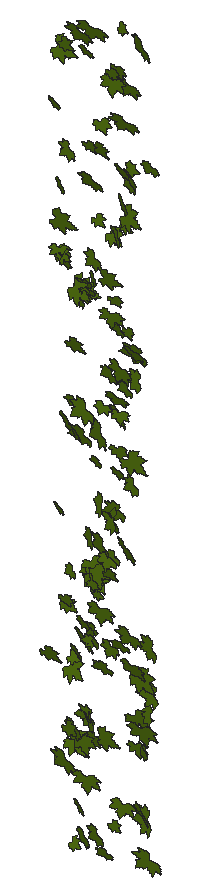
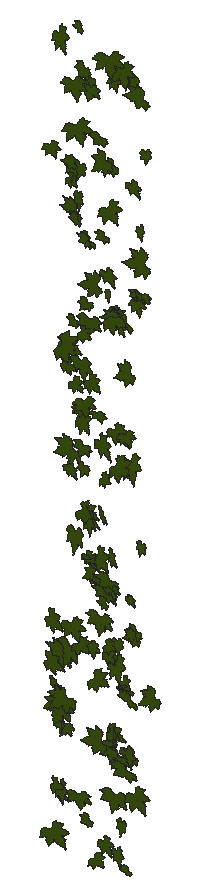
# SketchUp Ruby script. Lengths in inches.
U = 1.inch
M = Sketchup.active_model
def pt(a) = Geom::Point3d.new(a.map { |v| v * U })
def face(e, loops, mat)
  f = e.add_face(loops[0].map { |a| pt(a) })
  loops[1..].each { |l| e.add_face(l.map { |a| pt(a) }).erase! }
  f.material = f.back_material = mat if mat
  f
end
# faces: each face lists its corners as indices into pts; further lists are holes
def faces(e, pts, list, mat = nil) = list.each { |f| face(e, (f[0].is_a?(Array) ? f : [f]).map { |l| l.map { |i| pts[i] } }, mat) }
# xy, xz, yz: faces in a plane at the given z, y or x. An outline is a flat list of corners, or four numbers for a rectangle; further outlines are holes
def ring(l) = l.size == 4 ? [[l[0], l[1]], [l[2], l[1]], [l[2], l[3]], [l[0], l[3]]] : l.each_slice(2).to_a
def flat(e, list, mat, &to3) = list.each { |f| face(e, (f[0].is_a?(Array) ? f : [f]).map { |l| ring(l).map { |u, v| to3.(u, v) } }, mat) }
def xy(e, z, list, mat = nil) = flat(e, list, mat) { |x, y| [x, y, z] }
def xz(e, y, list, mat = nil) = flat(e, list, mat) { |x, z| [x, y, z] }
def yz(e, x, list, mat = nil) = flat(e, list, mat) { |y, z| [x, y, z] }
def lines(e, pts, list) = list.each { |a, b| e.add_line(pt(pts[a]), pt(pts[b])) }
# prism: a flat outline (further loops are holes) pulled along v
def prism(e, loops, v, mat = nil)
  f = face(e, loops, mat); d = Geom::Vector3d.new(v.map { |x| x * U })
  f.pushpull(f.normal.samedirection?(d) ? d.length : -d.length)
end
def box(e, o, s, mat = nil) = prism(e, [[o, [o[0] + s[0], o[1], o[2]], [o[0] + s[0], o[1] + s[1], o[2]], [o[0], o[1] + s[1], o[2]]]], [0, 0, s[2]], mat)
def at(x, y, z, deg = 0) = Geom::Transformation.translation(pt([x, y, z])) * Geom::Transformation.rotation(ORIGIN, Z_AXIS, deg.degrees)
def axes(o, x, y, z) = Geom::Transformation.new([*x, 0, *y, 0, *z, 0, *pt(o).to_a, 1])
def part(name) = M.definitions.add(name)
# library, detail: a bought-in or finely detailed component or shape, given as its bounding box
def library(name, o, s) = part(name).tap { |d| box(d.entities, o, s) }
def detail(e, o, s) = box(e.add_group.entities, o, s)
def put(e, d, t, mat = nil) = e.add_instance(d, t).tap { |i| i.material = mat if mat }
def group(e, t, mat = nil) = e.add_group.tap { |g| g.transformation = t; g.material = mat if mat }.entities
root = M.entities
M.materials.add("[Vegetation Blur 03]").color = [83, 114, 18]
c1 = part("ivy")
xy(c1.entities,0,[[0.782,0,0.786,0,0.787,0.005,0.789,0.009,0.821,0.072,0.875,0.147,1.001,0.272,1.073,0.331,1.137,0.363,1.178,0.379,1.223,0.384,1.272,0.383,1.311,0.374,1.36,0.355,1.399,0.334,1.491,0.285,1.541,0.244,1.583,0.199,1.617,0.15,1.64,0.128,1.662,0.115,1.717,0.105,1.745,0.093,1.784,0.054,1.819,0.057,1.854,0.064,1.882,0.075,1.896,0.074,1.91,0.071,1.937,0.063,1.964,0.053,1.99,0.038,2.016,0.015,2.034,0.002,2.04,0,2.038,0.003,2.036,0.007,2.033,0.038,2.036,0.068,2.045,0.1,2.055,0.116,2.064,0.123,2.077,0.129,2.088,0.129,2.106,0.132,2.118,0.13,2.179,0.132,2.207,0.133,2.225,0.133,2.242,0.138,2.22,0.162,2.207,0.186,2.206,0.213,2.212,0.236,2.228,0.262,2.247,0.274,2.298,0.283,2.355,0.294,2.37,0.296,2.376,0.295,2.377,0.3,2.377,0.303,2.385,0.329,2.411,0.37,2.426,0.392,2.449,0.407,2.511,0.426,2.561,0.444,2.619,0.466,2.589,0.469,2.561,0.476,2.501,0.5,2.449,0.516,2.424,0.523,2.401,0.535,2.377,0.556,2.372,0.568,2.36,0.575,2.268,0.586,2.225,0.592,2.207,0.599,2.194,0.61,2.143,0.65,2.13,0.664,2.122,0.682,2.123,0.7,2.13,0.719,2.148,0.75,2.17,0.781,2.195,0.807,2.221,0.828,2.284,0.874,2.291,0.88,2.288,0.887,2.276,0.9,2.267,0.916,2.265,0.933,2.273,0.967,2.292,1.002,2.313,1.03,2.334,1.054,2.348,1.067,2.358,1.074,2.363,1.076,2.362,1.081,2.35,1.094,2.347,1.11,2.35,1.143,2.359,1.18,2.385,1.254,2.415,1.324,2.448,1.393,2.45,1.4,2.446,1.398,2.44,1.394,2.427,1.383,2.402,1.36,2.376,1.339,2.345,1.324,2.305,1.309,2.282,1.303,2.273,1.306,2.245,1.294,2.212,1.287,2.187,1.291,2.163,1.301,2.142,1.316,2.134,1.327,2.124,1.325,2.09,1.292,2.053,1.259,2.014,1.234,1.973,1.215,1.954,1.21,1.931,1.208,1.909,1.212,1.893,1.22,1.879,1.233,1.872,1.248,1.867,1.281,1.864,1.319,1.821,1.258,1.773,1.197,1.726,1.141,1.698,1.121,1.679,1.116,1.666,1.117,1.647,1.122,1.632,1.129,1.62,1.141,1.617,1.154,1.617,1.219,1.621,1.254,1.623,1.268,1.623,1.281,1.618,1.314,1.606,1.346,1.603,1.375,1.607,1.403,1.603,1.467,1.599,1.499,1.605,1.525,1.614,1.552,1.629,1.577,1.635,1.589,1.629,1.587,1.618,1.582,1.596,1.566,1.581,1.556,1.568,1.552,1.557,1.55,1.545,1.553,1.531,1.562,1.522,1.572,1.504,1.591,1.486,1.611,1.474,1.631,1.457,1.666,1.455,1.684,1.457,1.698,1.452,1.715,1.444,1.728,1.424,1.754,1.419,1.772,1.423,1.786,1.434,1.819,1.444,1.848,1.446,1.855,1.44,1.861,1.43,1.867,1.386,1.904,1.349,1.948,1.326,1.973,1.31,1.995,1.288,2.048,1.284,2.153,1.287,2.254,1.284,2.255,1.282,2.253,1.278,2.247,1.274,2.237,1.266,2.216,1.226,2.125,1.208,2.076,1.184,2.033,1.155,1.984,1.135,1.942,1.111,1.899,1.083,1.861,1.053,1.85,1.059,1.83,1.061,1.809,1.056,1.79,1.049,1.767,1.04,1.749,1.018,1.733,0.994,1.726,0.942,1.734,0.95,1.6875,0.944,1.645,0.932,1.608,0.911,1.585,0.881,1.58,0.854,1.582,0.828,1.588,0.785,1.618,0.773,1.625,0.775,1.614,0.779,1.598,0.796,1.502,0.818,1.402,0.861,1.283,0.882,1.224,0.894,1.174,0.892,1.148,0.886,1.123,0.881,1.107,0.872,1.099,0.849,1.094,0.818,1.092,0.789,1.098,0.762,1.107,0.753,1.113,0.721,1.139,0.698,1.163,0.678,1.194,0.665,1.224,0.628,1.28,0.612,1.312,0.606,1.327,0.606,1.314,0.599,1.282,0.594,1.267,0.581,1.256,0.544,1.245,0.512,1.244,0.473,1.249,0.444,1.256,0.382,1.288,0.339,1.306,0.324,1.316,0.317,1.324,0.309,1.326,0.27,1.314,0.227,1.313,0.185,1.3125,0.152,1.317,0.122,1.328,0.092,1.345,0.073,1.353,0.079,1.338,0.092,1.308,0.117,1.249,0.13,1.215,0.139,1.164,0.147,1.148,0.157,1.136,0.163,1.122,0.174,1.086,0.177,1.067,0.182,1.054,0.186,1.043,0.191,1.038,0.211,1.028,0.237,1.005,0.25,0.974,0.253,0.96,0.25,0.944,0.242,0.914,0.243,0.906,0.249,0.902,0.26,0.894,0.289,0.88,0.307,0.873,0.322,0.862,0.364,0.799,0.403,0.738,0.431,0.709,0.439,0.691,0.441,0.678,0.4375,0.66,0.428,0.645,0.394,0.623,0.303,0.594,0.255,0.581,0.214,0.577,0.179,0.573,0.173,0.568,0.175,0.561,0.167,0.55,0.141,0.523,0.113,0.503,0.077,0.49,0.045,0.486,0.026,0.485,0.019,0.486,0.011,0.483,0,0.471,0.014,0.467,0.044,0.455,0.058,0.447,0.07,0.438,0.097,0.411,0.125,0.394,0.158,0.377,0.174,0.366,0.182,0.359,0.185,0.361,0.242,0.331,0.253,0.316,0.258,0.303,0.262,0.283,0.274,0.278,0.308,0.274,0.341,0.252,0.366,0.226,0.366,0.222,0.37,0.22,0.38,0.221,0.395,0.221,0.425,0.216,0.45,0.207,0.465,0.192,0.473,0.178,0.484,0.15,0.489,0.116,0.483,0.089,0.468,0.058,0.45,0.035,0.435,0.018,0.429,0.011,0.434,0.012,0.438,0.014,0.469,0.019,0.542,0.016,0.581,0.015,0.612,0.027,0.68,0.055,0.696,0.057,0.712,0.052,0.73,0.045,0.741,0.036,0.766,0.014]])
put(root,c1,axes([17.67,173.7,15.6],[0.33482,-0.12296,0.29954],[0.37174,0.13576,-0.26801],[0.00918,-1.01326,-0.07226]),"[Vegetation Blur 03]")
put(root,c1,axes([18.34,173.7,44.47],[0.29211,-0.05666,-0.12031],[-0.1385,0.15286,-0.23529],[-0.05752,-0.65573,-0.04445]),"[Vegetation Blur 03]")
put(root,c1,axes([18.82,173.7,40.44],[0.23798,-0.09799,-0.20106],[-0.2294,0.19812,-0.19604],[-0.10166,-0.67644,-0.02829]),"[Vegetation Blur 03]")
put(root,c1,axes([18.85,173.7,11.16],[0.44315,0.00145,-0.39097],[-0.47521,0.17095,-0.35867],[-0.06051,-1.33197,-0.04646]),"[Vegetation Blur 03]")
put(root,c1,axes([18.59,173.7,23.7],[0.31001,-0.14403,-0.03677],[-0.03088,0.13304,-0.25536],[-0.0773,-0.63077,-0.04546]),"[Vegetation Blur 03]")
put(root,c1,axes([18.78,173.7,36.65],[0.35037,-0.01321,-0.20166],[-0.24181,0.16441,-0.28153],[-0.0512,-0.86678,-0.05033]),"[Vegetation Blur 03]")
put(root,c1,axes([18.3,173.7,36.83],[0.4392,0.07424,0.06802],[0.08567,-0.05755,-0.35857],[0.03015,-0.91812,0.02798]),"[Vegetation Blur 03]")
put(root,c1,axes([19.05,173.7,28.47],[0.46716,-0.062,-0.38996],[-0.44887,0.42109,-0.3687],[-0.16652,-1.30905,-0.10013]),"[Vegetation Blur 03]")
put(root,c1,axes([18.33,173.7,46.5],[0.13182,0.09274,0.49871],[0.61259,0.00582,-0.10802],[0.01227,-1.28635,0.03547]),"[Vegetation Blur 03]")
put(root,c1,axes([18.61,173.7,36.14],[0.09631,0.08819,0.32844],[0.40359,-0.08421,-0.07527],[-0.03009,-0.84734,0.04167]),"[Vegetation Blur 03]")
put(root,c1,axes([18.33,173.7,37.74],[0.17934,-0.09894,0.51265],[0.6295,0.08025,-0.14425],[0.02442,-1.34184,-0.04643]),"[Vegetation Blur 03]")
put(root,c1,axes([19.26,173.7,42.62],[0.34594,-0.11487,-0.25725],[-0.31497,0.04827,-0.28551],[-0.05712,-0.96184,0.01639]),"[Vegetation Blur 03]")
put(root,c1,axes([18.78,173.7,18.89],[0.3213,-0.06644,0.14929],[0.18483,0.03966,-0.26218],[-0.01845,-0.75978,-0.02674]),"[Vegetation Blur 03]")
put(root,c1,axes([18.79,173.7,47.24],[0.18668,-0.06069,0.28857],[0.35478,0.02187,-0.15215],[-0.00434,-0.8225,-0.02534]),"[Vegetation Blur 03]")
put(root,c1,axes([18.86,173.7,18.36],[0.19136,0.01715,0.31471],[0.38568,-0.01715,-0.15606],[-0.00376,-0.88569,0.00911]),"[Vegetation Blur 03]")
put(root,c1,axes([19.41,173.7,29.49],[0.29858,0.09929,-0.17499],[-0.21887,0.06675,-0.24279],[0.01995,-0.75348,-0.04457]),"[Vegetation Blur 03]")
put(root,c1,axes([19.55,173.7,20.86],[0.2154,-0.10325,-0.19292],[-0.23671,0.04089,-0.17948],[-0.04859,-0.65681,0.01915]),"[Vegetation Blur 03]")
put(root,c1,axes([19.8,173.7,16.61],[0.12889,0.05373,-0.25764],[-0.31029,0.16238,-0.09807],[-0.06367,-0.68262,-0.04361]),"[Vegetation Blur 03]")
put(root,c1,axes([19.43,173.7,12.93],[0.42245,-0.13873,-0.23601],[-0.28027,0.15555,-0.34853],[-0.09809,-1.04193,-0.02061]),"[Vegetation Blur 03]")
put(root,c1,axes([19.27,173.7,15.65],[0.07011,0.12287,0.23012],[0.28735,0.0166,-0.05971],[0.0224,-0.59768,0.04565]),"[Vegetation Blur 03]")
put(root,c1,axes([18.99,173.7,12.1],[0.22931,-0.05412,0.29769],[0.36487,-0.02596,-0.18795],[-0.02469,-0.88622,-0.01267]),"[Vegetation Blur 03]")
put(root,c1,axes([20.1,173.7,28.09],[0.19085,0.16255,-0.44019],[-0.54494,0.0863,-0.15236],[-0.01363,-1.17416,-0.07214]),"[Vegetation Blur 03]")
put(root,c1,axes([19.43,173.7,48.74],[0.51903,0.05216,-0.26245],[-0.32095,0.20906,-0.41624],[-0.03231,-1.23893,-0.08129]),"[Vegetation Blur 03]")
put(root,c1,axes([19.39,173.7,6.15],[0.08845,0.08211,0.23234],[0.28731,-0.04554,-0.07032],[-0.00952,-0.61175,0.03642]),"[Vegetation Blur 03]")
put(root,c1,axes([18.99,173.7,14.93],[0.19869,0.16598,0.44202],[0.5434,-0.20587,-0.15053],[-0.06748,-1.16914,0.08926]),"[Vegetation Blur 03]")
put(root,c1,axes([18.98,173.7,11.34],[0.3778,0.16016,0.36511],[0.45377,-0.08873,-0.30663],[0.01685,-1.20168,0.0713]),"[Vegetation Blur 03]")
put(root,c1,axes([20.16,173.7,35.13],[0.17466,-0.11177,-0.29584],[-0.34642,0.21964,-0.14928],[-0.11976,-0.79834,0.00035]),"[Vegetation Blur 03]")
put(root,c1,axes([19.17,173.7,32],[0.29936,-0.14494,0.31849],[0.3965,0.0953,-0.24142],[-0.00556,-1.00761,-0.06865]),"[Vegetation Blur 03]")
put(root,c1,axes([19.95,173.7,17.64],[0.40831,-0.04926,-0.36189],[-0.41615,0.39004,-0.3211],[-0.15494,-1.17746,-0.09123]),"[Vegetation Blur 03]")
put(root,c1,axes([20.57,173.7,35.72],[0.10531,0.2061,-0.4524],[-0.56328,0.04564,-0.08406],[-0.00345,-1.16018,-0.08367]),"[Vegetation Blur 03]")
put(root,c1,axes([19.75,173.7,8.83],[0.35108,-0.18402,-0.07774],[-0.07773,0.15757,-0.29247],[-0.10502,-0.7318,-0.04343]),"[Vegetation Blur 03]")
put(root,c1,axes([20.125,173.7,29.68],[0.41789,-0.06408,-0.38347],[-0.47,0.02266,-0.34176],[-0.02893,-1.29377,0.01301]),"[Vegetation Blur 03]")
put(root,c1,axes([19.28,173.7,34.47],[0.16468,0.13945,0.51477],[0.63081,-0.17776,-0.12684],[-0.06707,-1.32961,0.07095]),"[Vegetation Blur 03]")
put(root,c1,axes([20.07,173.7,7.47],[0.35757,-0.14861,-0.22341],[-0.2596,0.18993,-0.29662],[-0.11295,-0.907,-0.02551]),"[Vegetation Blur 03]")
put(root,c1,axes([19.97,173.7,18.33],[0.32932,-0.07979,-0.11263],[-0.13041,0.12861,-0.26832],[-0.05951,-0.72344,-0.03528]),"[Vegetation Blur 03]")
put(root,c1,axes([20.19,173.7,47.77],[0.26625,0.02526,-0.1848],[-0.22371,0.14694,-0.21152],[-0.03714,-0.70407,-0.05077]),"[Vegetation Blur 03]")
put(root,c1,axes([20.67,173.7,13.84],[0.13243,-0.0083,-0.40164],[-0.49158,0.04791,-0.10811],[-0.02353,-1.04762,-0.00176]),"[Vegetation Blur 03]")
put(root,c1,axes([20.57,173.7,35.3125],[0.07838,0.01913,-0.25028],[-0.30675,-0.00782,-0.06408],[0.00599,-0.6513,-0.00658]),"[Vegetation Blur 03]")
put(root,c1,axes([20.39,173.7,41.28],[0.33022,0.14446,-0.3444],[-0.42741,0.15711,-0.26261],[-0.01782,-1.09139,-0.08339]),"[Vegetation Blur 03]")
put(root,c1,axes([20.03,173.7,35.2],[0.33133,0.03179,-0.00697],[-0.01113,0.11989,-0.26643],[0.0137,-0.67142,-0.0479]),"[Vegetation Blur 03]")
put(root,c1,axes([20.72,173.7,22.95],[0.13696,-0.09293,-0.32969],[-0.38837,0.22901,-0.11762],[-0.11998,-0.84735,0.00437]),"[Vegetation Blur 03]")
put(root,c1,axes([20.25,173.7,13.54],[0.33215,-0.12492,-0.16924],[-0.19211,0.18741,-0.2729],[-0.09889,-0.78367,-0.03828]),"[Vegetation Blur 03]")
put(root,c1,axes([19.63,173.7,10.25],[0.6157,0.01002,0.02515],[0.03061,0.04996,-0.50212],[0.00607,-1.26758,-0.01959]),"[Vegetation Blur 03]")
put(root,c1,axes([19.48,173.7,12.03],[0.55674,-0.05035,0.19483],[0.23814,-0.03752,-0.45478],[-0.02967,-1.24598,0.00582]),"[Vegetation Blur 03]")
put(root,c1,axes([19.97,173.7,49.05],[0.59461,0.12109,-0.18026],[-0.22736,0.18289,-0.48022],[0.02354,-1.29241,-0.08484]),"[Vegetation Blur 03]")
put(root,c1,axes([19.83,173.7,34.58],[0.10294,0.13872,0.40661],[0.50198,0.02961,-0.08624],[0.02785,-1.04645,0.05146]),"[Vegetation Blur 03]")
put(root,c1,axes([20.84,173.7,17.54],[0.04662,-0.02211,-0.24119],[-0.29524,-0.03871,-0.03745],[0.01692,-0.61444,0.01104]),"[Vegetation Blur 03]")
put(root,c1,axes([20.76,173.7,17.9],[0.21141,-0.03642,-0.34067],[-0.40654,0.204,-0.17147],[-0.09632,-0.94099,-0.02399]),"[Vegetation Blur 03]")
put(root,c1,axes([20.86,173.7,18.15],[0.07372,0.06524,-0.26494],[-0.3259,0.04312,-0.05873],[-0.01352,-0.68368,-0.02899]),"[Vegetation Blur 03]")
put(root,c1,axes([20.55,173.7,13.72],[0.32192,-0.21102,-0.29136],[-0.33943,0.22769,-0.27574],[-0.15085,-0.96265,-0.00135]),"[Vegetation Blur 03]")
put(root,c1,axes([20.6,173.7,20.78],[0.30881,-0.07275,-0.21101],[-0.25864,0.02403,-0.25343],[-0.03462,-0.82843,0.01118]),"[Vegetation Blur 03]")
put(root,c1,axes([20.14,173.7,42.69],[0.29342,-0.08692,0.17033],[0.21238,0.06683,-0.23833],[-0.01533,-0.73794,-0.04165]),"[Vegetation Blur 03]")
put(root,c1,axes([21.1,173.7,26.76],[0.04516,0.08728,-0.24004],[-0.29622,0.06188,-0.03358],[-0.02362,-0.6092,-0.0378]),"[Vegetation Blur 03]")
put(root,c1,axes([20.69,173.7,37.52],[0.38178,-0.11889,-0.25625],[-0.31299,0.05919,-0.31491],[-0.06294,-1.01546,0.01165]),"[Vegetation Blur 03]")
put(root,c1,axes([20.85,173.7,7.86],[0.3336,-0.07994,-0.30777],[-0.37102,0.14358,-0.27372],[-0.07791,-1.02608,-0.01433]),"[Vegetation Blur 03]")
put(root,c1,axes([20.76,173.7,36.32],[0.23472,-0.16453,-0.13977],[-0.15775,0.13898,-0.20218],[-0.10411,-0.58153,-0.00877]),"[Vegetation Blur 03]")
put(root,c1,axes([20.07,173.7,21.02],[0.386,0.08915,0.27036],[0.33331,-0.03157,-0.31533],[0.02283,-1.04625,0.03255]),"[Vegetation Blur 03]")
put(root,c1,axes([20.17,173.7,12.09],[0.30498,-0.11066,0.28031],[0.34736,0.05892,-0.24807],[-0.01408,-0.94337,-0.04838]),"[Vegetation Blur 03]")
put(root,c1,axes([21.09,173.7,28.82],[0.38094,-0.16652,-0.42659],[-0.51102,0.22607,-0.31784],[-0.13644,-1.3116,-0.00062]),"[Vegetation Blur 03]")
put(root,c1,axes([21.22,173.7,22.9375],[0.2944,-0.05147,-0.44172],[-0.52796,0.2576,-0.2391],[-0.12176,-1.24142,-0.0313]),"[Vegetation Blur 03]")
put(root,c1,axes([21.41,173.7,24.95],[0.09708,-0.16375,-0.35064],[-0.41312,0.26056,-0.09533],[-0.14231,-0.86813,0.03753]),"[Vegetation Blur 03]")
put(root,c1,axes([21.4375,173.7,16.41],[0.11047,0.20453,-0.35161],[-0.44126,-0.0065,-0.09294],[0.02783,-0.9152,-0.07792]),"[Vegetation Blur 03]")
put(root,c1,axes([20.01,173.7,20.8125],[0.58138,0.04851,0.24502],[0.30111,-0.07156,-0.47365],[0.00495,-1.34457,0.03405]),"[Vegetation Blur 03]")
put(root,c1,axes([20.67,173.7,38.86],[0.2013,0.04338,0.20783],[0.25534,-0.0094,-0.16443],[0.00948,-0.6679,0.01581]),"[Vegetation Blur 03]")
put(root,c1,axes([20.37,173.7,20.17],[0.3314,0.11464,0.31783],[0.39311,-0.13672,-0.26526],[-0.0151,-1.04335,0.06968]),"[Vegetation Blur 03]")
put(root,c1,axes([20.82,173.7,19.56],[0.07858,-0.01385,0.24493],[0.29907,-0.05144,-0.06436],[-0.02588,-0.6363,-0.00013]),"[Vegetation Blur 03]")
put(root,c1,axes([21.39,173.7,6.8125],[0.1696,0.1381,-0.24942],[-0.31204,0.02191,-0.13942],[0.02307,-0.7189,-0.05216]),"[Vegetation Blur 03]")
put(root,c1,axes([20.54,173.7,19.3],[0.62015,-0.02976,-0.03519],[-0.04222,0.07375,-0.50547],[-0.01689,-1.27709,-0.02837]),"[Vegetation Blur 03]")
put(root,c1,axes([20.4375,173.7,42.72],[0.41952,-0.13561,0.24997],[0.31292,0.12999,-0.33871],[-0.01528,-1.06095,-0.07345]),"[Vegetation Blur 03]")
put(root,c1,axes([21.13,173.7,29.82],[0.33208,0.00162,-0.09351],[-0.114,-0.06757,-0.26985],[0.01145,-0.71971,0.02513]),"[Vegetation Blur 03]")
put(root,c1,axes([20.77,173.7,44.02],[0.3458,0.03513,0.16386],[0.2014,-0.03386,-0.28195],[0.00648,-0.82214,0.01861]),"[Vegetation Blur 03]")
put(root,c1,axes([21.71,173.7,31.74],[0.21346,0.05085,-0.33078],[-0.40485,0.09932,-0.17162],[-0.03132,-0.93739,-0.03613]),"[Vegetation Blur 03]")
put(root,c1,axes([22.24,173.7,24.7],[0.10352,-0.20906,-0.49577],[-0.59692,0.27823,-0.10147],[-0.15173,-1.23717,0.06096]),"[Vegetation Blur 03]")
put(root,c1,axes([20.85,173.7,12.02],[0.20638,-0.06433,0.46905],[0.57546,0.04752,-0.16762],[0.01121,-1.25569,-0.03037]),"[Vegetation Blur 03]")
put(root,c1,axes([21.23,173.7,22.04],[0.4452,0.01529,-0.01974],[-0.02317,-0.10578,-0.36101],[0.01016,-0.91136,0.04157]),"[Vegetation Blur 03]")
put(root,c1,axes([21.47,173.7,17.6875],[0.43906,-0.08807,-0.12908],[-0.15747,0.03053,-0.36003],[-0.0453,-0.95985,0.00039]),"[Vegetation Blur 03]")
put(root,c1,axes([21.19,173.7,34.61],[0.54749,0.01991,-0.01395],[-0.01748,0.04635,-0.4465],[0.00896,-1.12621,-0.01862]),"[Vegetation Blur 03]")
put(root,c1,axes([22.22,173.7,24.92],[0.16632,0.09986,-0.39596],[-0.48659,-0.03313,-0.13745],[0.03103,-1.05488,-0.03317]),"[Vegetation Blur 03]")
put(root,c1,axes([21.91,173.7,22.375],[0.23314,-0.02071,-0.23083],[-0.28282,0.0106,-0.19042],[-0.01038,-0.7542,0.00366]),"[Vegetation Blur 03]")
put(root,c1,axes([21.72,173.7,24.26],[0.37136,-0.15214,-0.22354],[-0.25515,0.22677,-0.30661],[-0.12403,-0.92207,-0.03852]),"[Vegetation Blur 03]")
put(root,c1,axes([22.13,173.7,29.78],[0.25339,0.01902,-0.3994],[-0.47391,0.29322,-0.19806],[-0.12245,-1.09547,-0.05995]),"[Vegetation Blur 03]")
put(root,c1,axes([21.33,173.7,20.9],[0.22705,-0.08947,0.23456],[0.29067,0.06726,-0.18337],[-0.00101,-0.75069,-0.04439]),"[Vegetation Blur 03]")
put(root,c1,axes([21.64,173.7,30.45],[0.41502,0.09791,-0.15811],[-0.19925,0.15826,-0.33295],[0.0098,-0.92912,-0.07337]),"[Vegetation Blur 03]")
put(root,c1,axes([21.18,173.7,35.78],[0.15315,-0.11376,0.42127],[0.51825,0.09795,-0.12133],[0.03021,-1.10363,-0.05419]),"[Vegetation Blur 03]")
put(root,c1,axes([22.17,173.7,39.02],[0.17953,-0.09504,-0.30608],[-0.36446,0.18198,-0.15128],[-0.09974,-0.83603,0.00186]),"[Vegetation Blur 03]")
put(root,c1,axes([22.28,173.7,34.08],[0.09179,0.09251,-0.29251],[-0.35994,0.08732,-0.07089],[-0.03033,-0.7563,-0.04396]),"[Vegetation Blur 03]")
put(root,c1,axes([21.29,173.7,46.68],[0.55862,-0.01173,0.01902],[0.02312,-0.03492,-0.45573],[-0.0064,-1.15001,0.01364]),"[Vegetation Blur 03]")
put(root,c1,axes([21.49,173.7,46.86],[0.27413,-0.06194,0.16545],[0.20434,0.02916,-0.2238],[-0.01572,-0.70099,-0.02393]),"[Vegetation Blur 03]")
put(root,c1,axes([22.24,173.7,17.8],[0.1902,0.17643,-0.26649],[-0.33646,0.03567,-0.15623],[0.02775,-0.7768,-0.0677]),"[Vegetation Blur 03]")
put(root,c1,axes([21.6,173.7,35.2],[0.28384,0.00263,0.11756],[0.14245,0.09199,-0.22943],[0.02136,-0.64851,-0.03207]),"[Vegetation Blur 03]")
put(root,c1,axes([21.44,173.7,38.24],[0.23996,0.10055,0.29847],[0.36879,-0.09254,-0.19259],[-0.01117,-0.89532,0.05342]),"[Vegetation Blur 03]")
put(root,c1,axes([21.64,173.7,8.02],[0.1988,-0.0106,0.20658],[0.25313,-0.00387,-0.16228],[-0.00466,-0.6623,-0.00236]),"[Vegetation Blur 03]")
put(root,c1,axes([22.01,173.7,44.93],[0.48948,0.16058,-0.27855],[-0.34964,0.16113,-0.39462],[0.01829,-1.21733,-0.08898]),"[Vegetation Blur 03]")
put(root,c1,axes([21.87,173.7,26.61],[0.33381,-0.09287,0.01816],[0.028,0.08748,-0.27236],[-0.04181,-0.68286,-0.03736]),"[Vegetation Blur 03]")
put(root,c1,axes([21.73,173.7,27.66],[0.39754,-0.01789,0.09307],[0.11433,0.03939,-0.32408],[-0.00307,-0.85015,-0.01697]),"[Vegetation Blur 03]")
put(root,c1,axes([21.87,173.7,29.57],[0.37993,0.04432,0.03279],[0.04106,-0.03097,-0.31026],[0.01982,-0.78558,0.01408]),"[Vegetation Blur 03]")
put(root,c1,axes([21.78,173.7,47.3125],[0.38821,-0.11193,0.10755],[0.13579,0.05066,-0.31818],[-0.04343,-0.84212,-0.03344]),"[Vegetation Blur 03]")
put(root,c1,axes([21.875,173.7,32.3],[0.58763,-0.14391,-0.14762],[-0.17735,0.08172,-0.48275],[-0.07846,-1.26257,-0.01442]),"[Vegetation Blur 03]")
put(root,c1,axes([21.91,173.7,9.64],[0.52025,0.05923,-0.06815],[-0.08303,-0.02209,-0.42521],[0.03012,-1.08405,0.00494]),"[Vegetation Blur 03]")
put(root,c1,axes([22.08,173.7,42.35],[0.38893,-0.1332,-0.05202],[-0.05011,0.16639,-0.31658],[-0.07577,-0.79377,-0.05763]),"[Vegetation Blur 03]")
put(root,c1,axes([22.67,173.7,31.25],[0.18993,0.03098,-0.27697],[-0.33885,0.07408,-0.15347],[-0.02412,-0.79685,-0.02503]),"[Vegetation Blur 03]")
put(root,c1,axes([22.34,173.7,40.88],[0.36908,-0.2283,-0.18774],[-0.2052,0.23015,-0.31272],[-0.15204,-0.86483,-0.03366]),"[Vegetation Blur 03]")
put(root,c1,axes([22.25,173.7,46.97],[0.53586,0.00327,-0.21137],[-0.25728,0.14717,-0.4341],[-0.0297,-1.21585,-0.05311]),"[Vegetation Blur 03]")
put(root,c1,axes([22.26,173.7,49.14],[0.05613,0.01305,0.23736],[0.28926,-0.0672,-0.04498],[-0.03088,-0.6058,0.0101]),"[Vegetation Blur 03]")
put(root,c1,axes([22.44,173.7,18.7],[0.47827,0.03325,-0.27343],[-0.33498,0.10885,-0.38819],[-0.01718,-1.19669,-0.04291]),"[Vegetation Blur 03]")
put(root,c1,axes([22.99,173.7,41.81],[0.1507,0.00007,-0.27274],[-0.3307,0.10871,-0.1217],[-0.04814,-0.74651,-0.01775]),"[Vegetation Blur 03]")
put(root,c1,axes([22.26,173.7,23.22],[0.58057,-0.26082,-0.16045],[-0.16911,0.27993,-0.47915],[-0.16161,-1.22989,-0.07503]),"[Vegetation Blur 03]")
put(root,c1,axes([23.4375,173.7,33.36],[0.08849,0.22325,-0.50781],[-0.6312,-0.01504,-0.0743],[0.02262,-1.29319,-0.0868]),"[Vegetation Blur 03]")
put(root,c1,axes([22.37,173.7,39.03],[0.11812,0.02268,0.27727],[0.33763,-0.09352,-0.0946],[-0.03936,-0.73423,0.02061]),"[Vegetation Blur 03]")
put(root,c1,axes([22.47,173.7,33.9],[0.26219,-0.05379,0.13773],[0.16863,-0.0189,-0.21498],[-0.02696,-0.64136,-0.00522]),"[Vegetation Blur 03]")
put(root,c1,axes([22.64,173.7,42.26],[0.41315,-0.18544,-0.14251],[-0.1576,0.18691,-0.3426],[-0.11735,-0.90388,-0.04161]),"[Vegetation Blur 03]")
put(root,c1,axes([23.01,173.7,26.61],[0.30292,-0.11557,-0.26319],[-0.32214,0.05514,-0.25077],[-0.05807,-0.90879,0.01825]),"[Vegetation Blur 03]")
put(root,c1,axes([22.64,173.7,41.93],[0.04916,0.02287,0.27993],[0.3427,0.03405,-0.04052],[0.01796,-0.71221,0.00705]),"[Vegetation Blur 03]")
put(root,c1,axes([22.59,173.7,33.14],[0.46406,-0.05319,-0.06714],[-0.07481,0.21257,-0.37089],[-0.04289,-0.94624,-0.07954]),"[Vegetation Blur 03]")
put(root,c1,axes([23.57,173.7,32.08],[0.07216,-0.07343,-0.39325],[-0.48158,0.07012,-0.06092],[-0.03906,-1.00014,0.0246]),"[Vegetation Blur 03]")
put(root,c1,axes([22.3,173.7,39.25],[0.15618,0.05581,0.47785],[0.58342,-0.13447,-0.12454],[-0.05625,-1.2397,0.03502]),"[Vegetation Blur 03]")
put(root,c1,axes([22.375,173.7,17.01],[0.64437,-0.16461,0.01325],[0.02704,0.17964,-0.52482],[-0.07702,-1.31419,-0.0734]),"[Vegetation Blur 03]")
put(root,c1,axes([22.23,173.7,26.86],[0.3615,0.01419,0.44771],[0.54841,0.02846,-0.29509],[0.01534,-1.35164,-0.00151]),"[Vegetation Blur 03]")
put(root,c1,axes([23.37,173.7,49.39],[0.37946,-0.0754,-0.40939],[-0.47883,0.34147,-0.30552],[-0.15388,-1.24846,-0.05884]),"[Vegetation Blur 03]")
put(root,c1,axes([22.75,173.7,12.78],[0.44477,-0.01678,0.0841],[0.10333,0.04659,-0.36253],[-0.00282,-0.93833,-0.0195]),"[Vegetation Blur 03]")
put(root,c1,axes([23.35,173.7,9.88],[0.41747,-0.18159,-0.28175],[-0.32214,0.27535,-0.34584],[-0.15229,-1.08022,-0.04079]),"[Vegetation Blur 03]")
put(root,c1,axes([22.51,173.7,13.94],[0.46309,-0.00814,0.32802],[0.3991,0.15897,-0.37467],[0.04767,-1.25175,-0.04972]),"[Vegetation Blur 03]")
put(root,c1,axes([23.55,173.7,13.0625],[0.30175,-0.15566,-0.18852],[-0.22184,0.13329,-0.25383],[-0.09933,-0.77056,-0.00582]),"[Vegetation Blur 03]")
put(root,c1,axes([24.04,173.7,9.9],[0.23881,-0.20013,-0.4704],[-0.57401,0.16163,-0.20491],[-0.11037,-1.27363,0.04791]),"[Vegetation Blur 03]")
put(root,c1,axes([22.74,173.7,13.81],[0.67064,-0.03297,0.06761],[0.08405,0.14038,-0.54453],[-0.00745,-1.38343,-0.05687]),"[Vegetation Blur 03]")
put(root,c1,axes([23.67,173.7,7.68],[0.46314,0.05825,-0.39602],[-0.48604,0.04033,-0.37767],[0.00535,-1.37976,-0.02776]),"[Vegetation Blur 03]")
put(root,c1,axes([24.18,173.7,18.65],[0.20411,-0.06117,-0.44075],[-0.53473,0.15542,-0.16833],[-0.08116,-1.17781,0.00068]),"[Vegetation Blur 03]")
put(root,c1,axes([22.78,173.7,15.9375],[0.4004,-0.01607,0.44585],[0.54595,-0.04146,-0.32681],[-0.02086,-1.39316,0.00458]),"[Vegetation Blur 03]")
put(root,c1,axes([24.26,173.7,15.05],[0.07522,-0.13511,-0.31021],[-0.37954,0.11629,-0.06927],[-0.06884,-0.78881,0.04292]),"[Vegetation Blur 03]")
put(root,c1,axes([24.42,173.7,16.33],[0.13923,-0.07198,-0.4584],[-0.56199,0.04465,-0.11479],[-0.02951,-1.18996,0.02342]),"[Vegetation Blur 03]")
put(root,c1,axes([23.83,173.7,43.09],[0.32097,0.04197,-0.19874],[-0.24426,0.07998,-0.2601],[-0.00735,-0.82521,-0.03532]),"[Vegetation Blur 03]")
